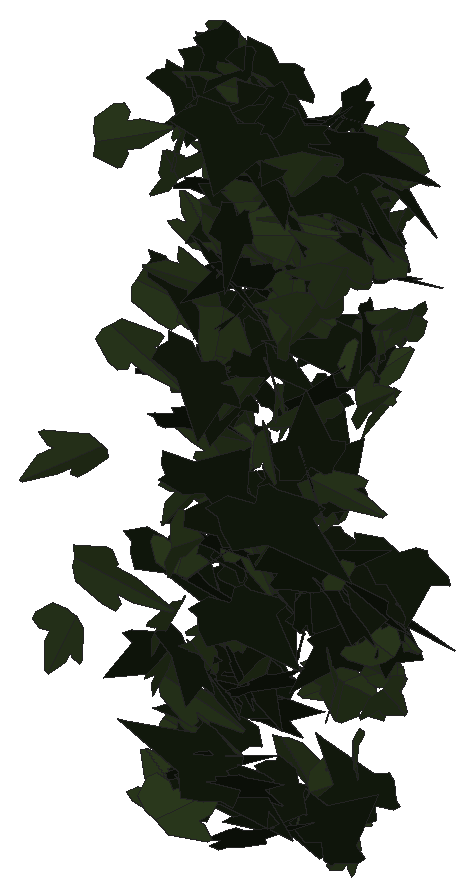
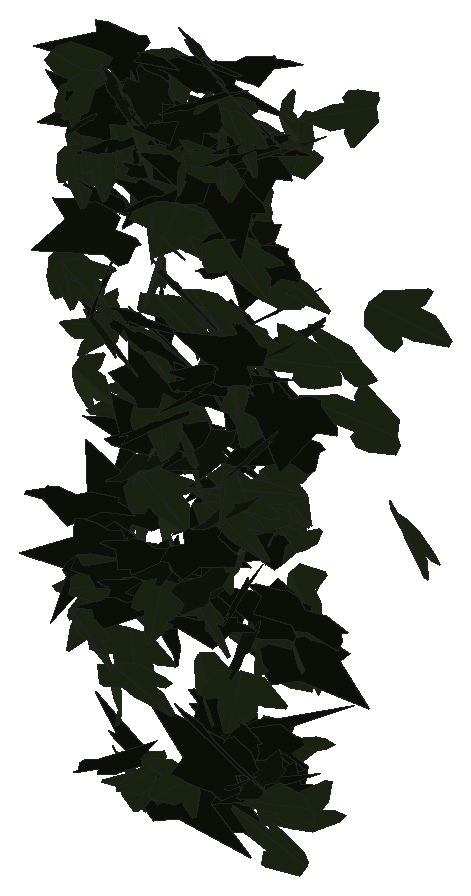
# SketchUp Ruby script. Lengths in millimetres.
U = 1.mm
M = Sketchup.active_model
def pt(a) = Geom::Point3d.new(a.map { |v| v * U })
def face(e, loops, mat)
  f = e.add_face(loops[0].map { |a| pt(a) })
  loops[1..].each { |l| e.add_face(l.map { |a| pt(a) }).erase! }
  f.material = f.back_material = mat if mat
  f
end
# faces: each face lists its corners as indices into pts; further lists are holes
def faces(e, pts, list, mat = nil) = list.each { |f| face(e, (f[0].is_a?(Array) ? f : [f]).map { |l| l.map { |i| pts[i] } }, mat) }
# xy, xz, yz: faces in a plane at the given z, y or x. An outline is a flat list of corners, or four numbers for a rectangle; further outlines are holes
def ring(l) = l.size == 4 ? [[l[0], l[1]], [l[2], l[1]], [l[2], l[3]], [l[0], l[3]]] : l.each_slice(2).to_a
def flat(e, list, mat, &to3) = list.each { |f| face(e, (f[0].is_a?(Array) ? f : [f]).map { |l| ring(l).map { |u, v| to3.(u, v) } }, mat) }
def xy(e, z, list, mat = nil) = flat(e, list, mat) { |x, y| [x, y, z] }
def xz(e, y, list, mat = nil) = flat(e, list, mat) { |x, z| [x, y, z] }
def yz(e, x, list, mat = nil) = flat(e, list, mat) { |y, z| [x, y, z] }
def lines(e, pts, list) = list.each { |a, b| e.add_line(pt(pts[a]), pt(pts[b])) }
# prism: a flat outline (further loops are holes) pulled along v
def prism(e, loops, v, mat = nil)
  f = face(e, loops, mat); d = Geom::Vector3d.new(v.map { |x| x * U })
  f.pushpull(f.normal.samedirection?(d) ? d.length : -d.length)
end
def box(e, o, s, mat = nil) = prism(e, [[o, [o[0] + s[0], o[1], o[2]], [o[0] + s[0], o[1] + s[1], o[2]], [o[0], o[1] + s[1], o[2]]]], [0, 0, s[2]], mat)
def at(x, y, z, deg = 0) = Geom::Transformation.translation(pt([x, y, z])) * Geom::Transformation.rotation(ORIGIN, Z_AXIS, deg.degrees)
def axes(o, x, y, z) = Geom::Transformation.new([*x, 0, *y, 0, *z, 0, *pt(o).to_a, 1])
def part(name) = M.definitions.add(name)
# library, detail: a bought-in or finely detailed component or shape, given as its bounding box
def library(name, o, s) = part(name).tap { |d| box(d.entities, o, s) }
def detail(e, o, s) = box(e.add_group.entities, o, s)
def put(e, d, t, mat = nil) = e.add_instance(d, t).tap { |i| i.material = mat if mat }
def group(e, t, mat = nil) = e.add_group.tap { |g| g.transformation = t; g.material = mat if mat }.entities
root = M.entities
M.materials.add("efeu1").color = [18, 25, 13]
M.materials.add("efeu2").color = [43, 57, 29]
c1 = part("ivyleaf_10")
p = [[0,12.8,-0.8],[-1.5,51.3,-10.9],[-4.9,51,-11.6],[-13.6,26.5,-7.3],[-13.2,15.9,-4.6],[-21.1,19.3,-7.2],
  [-29.5,16.3,-8.3],[-29.2,8.3,-6.2],[-19.7,-9.8,0.5],[-7.6,-13,4],[1,-12.2,5.8],[-0.4,51.1,-11.1],
  [-1.5,51.1,-10.9],[1,-12.4,5.9],[16.9,-12.4,3.5],[35.1,9.1,-5.1],[35,12.9,-6.1],[20.5,16.4,-4.9],
  [15.8,15,-3.8],[15.3,27.6,-7.1],[12.8,31.3,-7.8]]
faces(c1.entities,p,[[0,1,2,3,4,5,6,7,8,9,10],[11,12,0,13,14,15,16,17,18,19,20]],"efeu2")
c2 = part("ivyleaf_9")
p = [[39.1,54.8,31.7],[34.5,51.8,30.2],[-5.3,25.2,17.3],[-17.9,28.3,20.9],[-21.6,21.7,17],[-20.2,4.3,5.3],
  [-22.9,-0.3,2.5],[-17.1,-4,-0.6],[-2,-2.1,-1.2],[-0.7,-15.4,-10.1],[16.6,-22.3,-16.7],[21.1,-15.1,-12.5],
  [32.7,-10.7,-11],[46.1,-1.8,-6.6],[30.8,11.2,3.8]]
faces(c2.entities,p,[[0,1,2,3,4,5,6,7,8,9,10,11,12,13,14]],"efeu1")
put(root,c1,axes([3953.5,539.1,2196.3],[-0.45606,-0.68527,1.0215],[-0.63132,-0.96615,-0.72595],[2.25434,-0.4092,0.00335]))
put(root,c1,axes([3962.8,543.3,2043.3],[0.10342,-0.11388,1.24145],[2.36353,0.11376,-0.04392],[-0.20776,1.23742,0.11829]))
put(root,c1,axes([3909.3,561.1,1942.6],[1.68125,-0.86872,0.00346],[0.02052,0.00603,-1.23891],[1.65324,0.88336,0.01186]))
put(root,c2,axes([4068.5,665.6,1979.6],[0.04124,-0.63779,-0.98844],[0.0507,0.98862,-0.63733],[2.23826,-0.01064,0.03265]))
put(root,c1,axes([3895,656.8,2533.3],[0.07259,-0.06329,-1.22483],[1.29662,1.02007,-0.03149],[1.94096,-0.67907,0.06685]))
put(root,c2,axes([4052.5,691.4,2465.4],[-1.13162,0.14311,-0.93716],[1.64141,-0.37766,-0.60485],[-0.74915,-1.04364,0.09037]))
put(root,c2,axes([3994.6,700.6,2252.2],[-0.32323,-1.18488,0.38736],[-0.17032,-0.37834,-1.19653],[2.36639,-0.18908,-0.03321]))
put(root,c2,axes([4159.4,697.8,2148],[-0.25535,0.03617,1.01376],[-0.12285,-1.02082,0.02788],[1.9267,-0.06029,0.13614]))
put(root,c2,axes([4097.7,676.6,2113.9],[0.01123,-0.60676,-1.09595],[0.88147,1.01936,-0.56186],[2.21521,-0.40255,0.22913]))
put(root,c1,axes([3970.5,669.2,1675.2],[1.18753,0.16446,-0.9582],[1.172,0.81418,0.54075],[1.4318,-0.80286,0.3521]))
put(root,c2,axes([3966.8,711,1862.7],[-0.11397,-0.83575,0.70239],[-0.09588,-0.70059,-0.83789],[2.07554,-0.07825,-0.00014]))
put(root,c2,axes([4035,713.2,2571.4],[-1.13596,-0.94572,0.0103],[0.01136,-0.01595,-1.11824],[1.79996,-0.59674,0.01356]))
put(root,c1,axes([3948.4,708.4,1913.9],[0.23071,-1.13641,0.33175],[0.13111,-0.32615,-1.14239],[2.24927,0.13558,0.03256]))
put(root,c1,axes([3949,717.6,2475.8],[-0.50415,-0.86215,-0.63928],[-0.37326,-0.60849,0.9019],[-2.00833,0.32952,-0.00715]))
put(root,c1,axes([3948.5,712,1812.2],[0.14236,-0.098,1.21389],[2.30428,-0.12512,-0.08471],[0.24986,1.20974,0.08957]))
put(root,c1,axes([4190.8,709.8,2458.3],[-1.59618,-0.19977,0.58892],[-1.03173,-0.24965,-0.85669],[0.57996,-0.99393,0.09681]))
put(root,c2,axes([3992.8,704.3,1985],[0.50189,0.92298,0.30225],[-0.18514,-0.28652,0.95981],[1.83911,-0.28072,0.01414]))
put(root,c1,axes([4185.4,711.9,2432.1],[-1.3066,-0.76689,0.17145],[-0.19512,-0.13831,-1.02918],[1.4828,-0.69397,0.01565]))
put(root,c1,axes([4110.9,699.4,2073.7],[-0.11913,-0.98771,-0.66786],[0.13344,0.66457,-0.98942],[2.26527,-0.09109,0.02316]))
put(root,c1,axes([3940,714,1849.5],[0.2568,-1.17504,0.03833],[0.00608,-0.03822,-1.18276],[2.23752,0.13496,-0.00118]))
put(root,c1,axes([3871.8,712.3,2237.8],[1.0563,0.08963,0.93672],[1.77529,0.09088,-0.56138],[-0.23596,1.085,-0.03036]))
put(root,c2,axes([4117.5,694.3,2028.2],[0.38673,0.0841,1.23687],[2.17532,0.47271,-0.21991],[-0.91378,1.1609,-0.00006]))
put(root,c2,axes([4001.8,728.5,1715.6],[-0.69414,-1.1102,-0.37263],[-0.21997,-0.35426,1.16857],[-2.21789,0.3826,0.00073]))
put(root,c1,axes([4113.7,692.7,2334.9],[0.23097,0.0758,-1.11438],[0.23761,1.11299,0.0893],[2.11247,-0.13348,0.1118]))
put(root,c2,axes([3990.1,714.2,2080.1],[-1.10932,-0.03055,0.83181],[1.54238,-0.25252,0.5586],[0.36144,0.98381,0.16921]))
put(root,c1,axes([4138.1,723.1,2372.2],[-1.11874,-1.08665,0.27018],[-0.24108,-0.23865,-1.23545],[2.11739,-0.60131,0.00209]))
put(root,c1,axes([4185.8,699.1,1902.9],[0.38525,-0.55887,-1.09726],[-0.1788,1.10174,-0.57848],[2.33675,0.17644,0.13664]))
put(root,c1,axes([3958.5,697.5,2007.9],[0.02773,-0.40498,-1.16165],[0.39577,1.14583,-0.39685],[2.30766,-0.19165,0.08202]))
put(root,c2,axes([4068.5,700.4,1861.9],[0.97182,0.67719,0.56864],[0.59009,0.47784,-0.84747],[-1.5761,0.59645,0.03333]))
put(root,c1,axes([4054.8,736.4,2159.7],[0.47293,-0.25048,0.96234],[1.33711,-0.65777,-0.35262],[1.33937,0.74511,0.01222]))
put(root,c1,axes([3941.5,737.7,2536.9],[0.70975,-0.78141,0.76922],[0.69407,-0.67784,-0.86539],[1.96804,0.52086,0.02779]))
put(root,c2,axes([4165.7,746.5,1982.1],[-0.19574,-0.69461,0.89319],[0.21233,-0.89873,-0.68607],[2.14296,0.0256,0.14956]))
put(root,c2,axes([4030.4,722.8,2058.2],[-1.5828,0.55974,0.19008],[-0.30204,0.10464,-1.00247],[-1.08374,-0.84666,0.00177]))
put(root,c2,axes([4036.3,734.5,2378.4],[-0.27964,0.51781,-0.87248],[-0.03773,-0.88288,-0.52065],[-1.93057,-0.05775,0.13655]))
put(root,c1,axes([4032,732.8,2225.2],[-0.46898,-0.95582,0.27345],[-0.13208,-0.2645,-0.98707],[1.88749,-0.256,-0.00113]))
put(root,c1,axes([3986.1,733.5,2418.8],[0.08471,-0.20955,0.99847],[1.9016,-0.19306,-0.08506],[0.39247,0.98064,0.19662]))
put(root,c2,axes([3931.7,736.4,1846.1],[0.21674,0.29858,-0.99083],[-0.63281,-0.93341,-0.31949],[-1.86509,0.35139,-0.00674]))
put(root,c2,axes([4011.5,714.2,1707.4],[1.50908,0.55786,0.29525],[0.44153,0.18329,-0.96937],[-1.11716,0.82601,0.0157]))
put(root,c2,axes([4142.6,713.4,2170],[-1.68294,0.61344,-0.33012],[-0.53232,0.17594,1.07612],[1.21427,0.92734,0.01421]))
put(root,c2,axes([4041.8,752.3,2497.9],[-0.10021,-0.90569,0.67551],[0.45221,-0.67,-0.87977],[2.10226,0.10095,0.22144]))
put(root,c1,axes([4131.1,737.3,2547.4],[-1.06216,-0.86661,0.25518],[-0.27664,-0.20989,-1.03073],[1.69694,-0.57665,-0.00831]))
put(root,c1,axes([3944.9,719.4,1970.1],[0.62125,0.76329,-0.56949],[0.42362,0.52419,0.83016],[1.76228,-0.39509,0.00121]))
put(root,c1,axes([3964.5,723.6,1865.7],[-0.87576,-0.9413,-0.64512],[0.46835,0.59738,-1.04716],[2.12073,-0.52063,-0.03515]))
put(root,c1,axes([3954.2,748.1,2064.2],[-0.264,-1.04651,0.60457],[-0.14105,-0.60003,-1.05565],[2.29586,-0.1572,0.00466]))
put(root,c2,axes([3976.3,745.6,2366.7],[0.92675,-0.82806,0.32776],[0.27851,-0.29408,-0.96038],[1.67189,0.508,-0.0217]))
put(root,c1,axes([3978.4,744.7,2134.1],[-1.15558,0.06455,0.81247],[1.47221,-0.27349,0.59981],[0.48859,0.97672,0.11426]))
put(root,c1,axes([4152.6,728.8,2020.2],[1.45952,-0.41695,0.66634],[-1.04669,0.38051,0.87104],[-1.06885,-0.94198,0.05691]))
put(root,c1,axes([4095.5,740.5,2439.4],[1.21864,-0.81411,-0.13122],[-0.1254,0.11509,-1.03557],[1.56439,0.6434,0.01921]))
put(root,c1,axes([3968,735.6,2332.1],[-0.45998,0.05211,0.98861],[-1.88399,0.00032,-0.24202],[-0.02414,-1.01773,0.05054]))
put(root,c1,axes([4067.1,731.7,2433.4],[0.74237,-0.07838,-0.94898],[1.76944,0.25294,0.36126],[0.39159,-0.99435,0.1667]))
put(root,c1,axes([4058.2,754.4,2215.6],[-0.58744,0.37768,0.92115],[1.15732,-0.69208,0.48752],[1.50025,0.68177,-0.0154]))
put(root,c2,axes([4070.7,746.8,2593.4],[-1.58531,0.49418,-0.33539],[0.45174,-0.25427,-0.96413],[-1.04305,-0.86121,0.0922]))
put(root,c2,axes([3950.7,725.8,1702.5],[0.48371,0.7736,-0.6093],[0.23986,0.59854,0.81251],[1.85875,-0.27856,0.05372]))
put(root,c2,axes([3980.4,750.8,2204.1],[-1.5148,-0.23059,-0.56353],[1.05969,0.09972,-0.82721],[0.46898,-0.97012,0.04892]))
put(root,c2,axes([3984.6,738.2,1699.9],[-0.34655,-0.27365,-1.02257],[1.17235,0.81643,-0.32817],[1.63841,-0.64207,0.01853]))
put(root,c2,axes([4095.1,757,2572.2],[-1.6129,-0.6342,-0.07722],[0.09986,0.05876,-1.05838],[1.21181,-0.84895,-0.01557]))
put(root,c1,axes([4011.9,755,2009.1],[1.36658,-0.30645,0.80688],[1.44018,-0.28134,-0.78025],[0.79014,1.04283,0.02661]))
put(root,c1,axes([4018.3,741.9,2389.7],[-0.05518,-0.93369,-0.40921],[0.0848,0.40782,-0.93368],[1.93831,-0.04442,0.0292]))
put(root,c2,axes([4000.7,736.6,1619.8],[0.81016,0.88116,-0.3023],[0.25031,0.27219,0.97859],[1.75521,-0.44554,-0.00002]))
put(root,c1,axes([3925.2,750,1636.4],[1.02843,1.0486,0.35028],[-0.33649,-0.3029,1.17951],[2.07702,-0.56828,0.01765]))
put(root,c1,axes([4084.4,744,2450.3],[-1.39093,-0.35841,-0.61342],[1.05352,0.26436,-0.81398],[0.84755,-0.9168,0.00509]))
put(root,c2,axes([4066,773.8,2463.1],[0.04859,-0.91032,0.80064],[0.13213,-0.79841,-0.90999],[2.30349,0.065,0.03531]))
put(root,c2,axes([4074.1,758.7,2565.5],[-1.83403,0.05238,0.56183],[-1.06917,0.01546,-0.96499],[-0.10096,-1.11537,0.01301]))
put(root,c2,axes([3970.6,749.5,1650.7],[-1.55831,-0.63423,0.4677],[0.70388,0.28629,1.03569],[-1.32434,0.89844,0.00014]))
put(root,c2,axes([3971,748.9,1996.1],[1.92699,-0.01233,-0.06006],[-0.11401,0.01285,-1.0125],[0.02487,1.0142,0.0121]))
put(root,c1,axes([4045.2,740.9,2017],[-0.78325,0.56329,0.78885],[-0.84278,0.6531,-0.69737],[-1.64106,-0.60426,-0.01837]))
put(root,c2,axes([4007,764.4,2069.1],[0.31794,-0.9687,-0.45375],[-0.0926,0.4519,-0.98265],[2.03375,0.17201,0.0262]))
put(root,c2,axes([4124.7,759,2513.7],[-0.10012,-0.49736,-0.98113],[1.02595,0.84456,-0.45703],[1.82488,-0.5021,0.20311]))
put(root,c1,axes([3961.6,771.5,2266.6],[2.04598,-0.563,0.17863],[0.32051,-0.06341,-1.21333],[1.07749,1.08792,0.02172]))
put(root,c2,axes([3921.5,750.9,2138.8],[1.51379,0.4763,0.35874],[0.59959,0.1721,-0.927],[-0.96353,0.85541,-0.01324]))
put(root,c1,axes([4127.6,759.7,2116.8],[-0.99301,-0.24041,-0.78625],[1.42432,0.24674,-0.57207],[0.64798,-0.91079,0.05256]))
put(root,c2,axes([4145.5,756.5,2564.8],[0.48075,0.11841,-0.99049],[1.0605,0.83074,0.24142],[1.57471,-0.59561,0.13981]))
put(root,c2,axes([4140.8,783.3,1909.8],[-0.17794,0.32339,-1.06895],[0.56755,-1.02651,-0.33663],[-2.04831,-0.31252,-0.00041]))
put(root,c2,axes([3913.1,775.4,1911.4],[0.89855,-0.42368,0.70592],[1.1409,-0.38089,-0.62953],[1.07405,0.75905,0.07813]))
put(root,c2,axes([4117.1,769.5,1645.8],[-0.82484,0.76744,0.77397],[0.73898,-0.66955,0.88133],[1.93829,0.58185,-0.00665]))
put(root,c1,axes([4040.8,794.5,2388.6],[-0.00111,-0.21122,1.13229],[-0.12037,-1.13057,-0.21093],[2.18884,-0.06228,-0.01103]))
put(root,c2,axes([4134.4,787.4,1969.5],[2.07397,-0.28345,-0.41835],[0.77322,-0.09994,1.12597],[-0.57192,-1.16298,0.0052]))
put(root,c2,axes([3976,762.5,2499.1],[0.51319,0.98217,-0.04078],[-0.03108,-0.03781,-1.0185],[-1.87063,0.27008,0.00573]))
put(root,c2,axes([3887.1,790.5,2292.9],[0.13252,-0.96869,0.27036],[0.07949,-0.26799,-0.97094],[1.91241,0.07826,0.02162]))
put(root,c2,axes([3917.3,765.1,2191.8],[1.20879,0.83868,-0.24486],[-0.31172,-0.18307,-1.05185],[-1.63333,0.65562,0.01953]))
put(root,c1,axes([3948.4,773.4,2225.4],[1.29995,-0.65518,0.33657],[-0.47755,0.22459,0.9464],[-1.318,-0.72758,-0.01094]))
put(root,c2,axes([4166.6,798.5,1982],[-0.50155,-0.92701,0.44825],[-0.13821,-0.44481,-0.9626],[1.95483,-0.26929,0.04695]))
put(root,c1,axes([3941.4,772.5,2048.7],[-0.10233,-0.07689,-1.07137],[2.00959,0.193,-0.06684],[0.37502,-1.05522,0.06584]))
put(root,c2,axes([4013.8,761.7,2211],[-0.13756,0.46618,0.92228],[-0.42672,0.89543,-0.47018],[-1.91992,-0.23242,0.03842]))
put(root,c2,axes([3909.3,799.8,2535.7],[-0.63465,-0.89236,0.41066],[0.08578,-0.44712,-0.93499],[1.86758,-0.28271,0.1825]))
put(root,c2,axes([4126.9,795.4,2483.9],[0.47542,-0.14624,-1.14518],[2.12427,-0.2688,0.2778],[-0.56144,-1.14087,0.08134]))
put(root,c2,axes([4018.8,798.9,1913],[0.15359,-0.88599,0.51674],[0.25457,-0.50481,-0.88645],[1.93539,0.13671,0.07559]))
put(root,c2,axes([4053.2,800.8,1682],[-0.54873,-0.7516,0.52577],[-0.38099,-0.48629,-0.80494],[1.70363,-0.35084,-0.01066]))
put(root,c1,axes([4145.2,781.7,1646.1],[1.09834,-0.74826,-0.2803],[-0.31591,0.22596,-0.94494],[1.48756,0.60046,0.00629]))
put(root,c1,axes([3953.9,777.5,2187.9],[-1.15627,-0.84557,-0.34477],[0.3323,0.2989,-1.04074],[1.70585,-0.63137,-0.03096]))
put(root,c2,axes([3879.1,787.1,1942.1],[-0.67637,-0.36584,-0.94495],[1.60956,0.4445,-0.49016],[1.06228,-0.90645,0.14102]))
put(root,c1,axes([4096.2,776.3,1988],[0.28382,-0.9081,-0.59435],[-0.26561,0.57891,-0.91952],[2.04841,0.20089,-0.03688]))
put(root,c2,axes([3983.9,785,2288.3],[-0.97506,0.78708,-0.34025],[0.39122,-0.27206,-0.93886],[-1.58435,-0.55157,-0.02243]))
put(root,c1,axes([4177.5,795.2,1907.3],[0.2415,0.91034,0.6083],[-0.20402,-0.5991,0.91893],[2.07375,-0.16496,0.01957]))
put(root,c2,axes([4087.7,778.2,2081.4],[-1.10349,-0.08986,0.99776],[1.8689,0.17722,0.5866],[-0.37741,1.14031,-0.01254]))
put(root,c2,axes([4114.9,796.2,2421.9],[-1.74984,-0.0918,-0.41817],[0.78731,0.06471,-0.92375],[0.20991,-1.00798,-0.02122]))
put(root,c2,axes([3966.6,806.4,2529.1],[-1.20519,-0.47169,0.62719],[-0.99407,-0.34815,-0.7892],[1.1147,-0.82046,-0.02569]))
put(root,c1,axes([3865.8,781.8,2266.7],[0.56961,0.1229,1.15898],[1.94317,0.54939,-0.32192],[-1.06968,1.06347,0.03237]))
put(root,c1,axes([4205.3,781.5,2435.1],[0.14544,-0.09058,-1.08147],[-1.61418,0.6714,-0.11617],[1.28862,0.85125,-0.02346]))
put(root,c2,axes([4127,795.9,1919.8],[0.17776,-0.00701,1.13133],[-2.05606,0.33653,0.09128],[-0.63938,-1.08415,0.02102]))
put(root,c1,axes([3995.9,794,2030.2],[1.42057,-0.17644,-0.64816],[-1.17648,0.19882,-0.76598],[0.50038,0.96836,0.03917]))
put(root,c1,axes([4093.4,813,2057.9],[-0.51625,0.49807,1.00316],[0.66044,-0.94399,0.56253],[2.02668,0.43449,0.07222]))
put(root,c2,axes([4084.7,781.8,1914.3],[-0.26341,-0.30348,0.95173],[0.92118,0.82013,0.33191],[-1.66313,0.50233,0.0331]))
put(root,c1,axes([4167.3,776.1,2231.5],[-0.07976,-0.2334,-1.06216],[0.47707,1.03225,-0.23672],[2.014,-0.25376,0.01401]))
put(root,c2,axes([4149.1,805.6,2495.8],[-1.76884,0.07374,0.34309],[-0.66787,-0.19852,-0.90795],[0.00222,-0.97061,0.21177]))
put(root,c2,axes([4068.4,798.9,1647.5],[0.20727,0.10245,-1.06024],[-1.6467,-0.6131,-0.14812],[-1.1824,0.87182,0.02042]))
put(root,c1,axes([4113.2,811.5,2476.4],[-0.24081,-0.87466,0.44632],[0.24827,-0.461,-0.86643],[1.85229,-0.05192,0.17416]))
put(root,c2,axes([4132.2,803.1,2502.2],[-0.51447,-0.84002,-0.601],[0.30844,0.57905,-0.88223],[1.94142,-0.3146,-0.0191]))
put(root,c2,axes([4099.6,805.5,2558.9],[-0.97737,0.70542,-0.56719],[0.35998,-0.55409,-0.86038],[-1.68468,-0.52765,0.14521]))
put(root,c1,axes([3963.1,804.7,2076.7],[0.78458,0.27682,0.93431],[-1.62873,-0.38233,0.49088],[0.88696,-0.94694,0.07493]))
put(root,c1,axes([3931.4,800.3,2348.3],[1.68288,0.19811,0.41243],[-0.7633,-0.09632,0.90614],[0.41911,-0.97092,-0.00574]))
put(root,c1,axes([4187.5,803.1,2516.9],[-0.96599,-0.88923,-0.05619],[0.06294,0.04582,-1.02387],[1.69459,-0.5086,0.006]))
put(root,c1,axes([3989.1,806.9,2558],[0.38613,0.05653,-1.1268],[-2.14688,-0.01,-0.20361],[-0.03781,1.14487,0.05386]))
put(root,c1,axes([4123.1,821.9,1746.2],[-0.05872,-0.04989,-0.93839],[0.28043,-0.92754,0.04447],[-1.76635,-0.1456,0.03826]))
put(root,c1,axes([4204.7,805.2,2555.2],[0.79101,0.00843,-0.96101],[-1.78295,0.2372,-0.40308],[0.40816,1.01981,0.1017]))
put(root,c2,axes([4081.6,820.5,2465.8],[-1.70627,-0.38907,0.27039],[-0.46015,-0.12199,-0.9772],[0.77549,-0.92844,0.01509]))
put(root,c1,axes([4079.3,815.4,2046.4],[-0.96799,-0.78369,0.47894],[-0.49743,-0.40134,-0.93427],[1.67572,-0.57184,-0.00067]))
put(root,c1,axes([4006.4,805.3,1828.6],[-0.00174,-1.13497,-0.31256],[0.0126,0.31255,-1.13496],[2.24045,-0.00264,0.00614]))
put(root,c1,axes([4089.7,807.4,1653.3],[1.12223,0.71891,0.1206],[0.14571,0.09319,-0.9298],[-1.37968,0.5946,-0.0001]))
put(root,c1,axes([4119.7,806,1826.2],[-1.97486,0.08011,0.28638],[-0.54346,0.02176,-1.04074],[-0.15798,-1.07622,0.00027]))
put(root,c1,axes([3879.6,804.7,1693.5],[0.45792,0.142,0.90249],[1.53877,0.40146,-0.27872],[-0.80961,0.84334,-0.01928]))
put(root,c2,axes([3931.5,831.1,1884.3],[0.62047,-0.31201,-1.00483],[1.42929,-0.66778,0.45101],[-1.4025,-0.81856,0.01508]))
put(root,c1,axes([4180.8,801.3,1845.6],[-0.39427,-0.80324,-0.61711],[0.44774,0.5745,-0.82676],[1.87508,-0.30608,0.06766]))
put(root,c1,axes([3873.9,819.5,1637.3],[0.5582,-0.21869,-1.04088],[1.67761,-0.55426,0.36483],[-1.13281,-0.92858,0.02738]))
put(root,c2,axes([4137.3,817,2253.6],[-1.29238,0.26166,0.62516],[-1.27255,-0.11437,-0.67841],[-0.2103,-0.91589,0.26332]))
put(root,c2,axes([3948,831.8,1938.3],[-0.17983,-0.23298,0.97162],[-0.68537,-0.90242,-0.25141],[1.7738,-0.3723,0.00136]))
put(root,c2,axes([3964.1,830.1,2382.7],[-1.09507,-0.5983,0.55719],[-0.76726,-0.38512,-0.82985],[1.35368,-0.70228,-0.01961]))
put(root,c2,axes([3948.5,820,2596],[-1.70653,0.26347,-0.4856],[0.83738,-0.21931,-0.93142],[-0.63591,-0.99585,0.07665]))
put(root,c2,axes([4063.8,816.1,2178.6],[1.1598,0.75277,0.57103],[-0.67247,-0.44863,0.96849],[1.66776,-0.70439,-0.00659]))
put(root,c1,axes([4021.6,805.3,2482.3],[-1.18871,0.31001,0.74421],[-1.38088,0.19425,-0.68985],[-0.66889,-0.95196,0.10159]))
put(root,c2,axes([3958.8,804.3,1803.2],[1.13108,-0.36565,-0.72433],[-1.15541,0.39529,-0.69766],[1.02453,0.84946,0.01287]))
put(root,c2,axes([4057.8,796.8,1852.4],[0.02798,0.06476,1.01548],[0.47963,0.98371,-0.06638],[-1.87625,0.25244,-0.00183]))
put(root,c2,axes([4000.2,833,2584.9],[-0.68689,-0.94212,0.23799],[-0.08422,-0.23767,-1.00799],[1.84744,-0.36112,0.04253]))
put(root,c2,axes([3973.1,803.8,2523.5],[1.26364,-0.11037,0.7519],[1.37575,0.39986,-0.57962],[-0.44638,0.91994,0.34215]))
put(root,c1,axes([3969.8,807.7,1973.1],[-0.4208,0.82835,-0.48441],[-0.3427,0.45246,0.8559],[1.79386,0.28075,0.04988]))
put(root,c2,axes([4158.9,824,2517.9],[1.03256,-0.88522,-0.02887],[-0.02657,0.0253,-1.03825],[1.68543,0.54272,0.00132]))
put(root,c2,axes([4168.4,824.1,2406.1],[-1.64668,0.22294,0.41903],[-0.81337,0.01313,-0.88942],[-0.39301,-0.96126,0.08503]))
put(root,c2,axes([3992.8,833.5,2547.9],[0.64634,-0.77266,0.60737],[0.6546,-0.50853,-0.83924],[1.75218,0.475,0.08949]))
put(root,c2,axes([4133,841.2,2296.1],[0.28206,-0.311,-1.0442],[1.42462,-0.73667,0.32565],[-1.50673,-0.75474,0.11243]))
put(root,c1,axes([4139.9,822.1,2518.7],[-1.62721,-0.49771,0.25526],[-0.4485,-0.10234,-0.98887],[0.96547,-0.88639,-0.02916]))
put(root,c1,axes([4071.3,808.7,2334.1],[0.39779,-0.71741,-0.74078],[0.29983,0.76919,-0.70047],[1.9396,0.02823,0.26021]))
put(root,c2,axes([4062,842.1,1941.5],[0.10819,-0.55444,0.98982],[0.38287,-0.97043,-0.55513],[2.12501,0.20308,0.04962]))
put(root,c1,axes([4138,816.8,1890.5],[-1.55676,-0.47877,-0.41518],[0.69427,0.1986,-0.94771],[0.98622,-0.89555,0.01179]))
put(root,c1,axes([3978.2,822.4,2405.1],[1.16531,-0.02497,-0.8142],[-1.53435,0.12723,-0.61017],[0.22193,1.01076,0.05669]))
put(root,c2,axes([3933.3,843,1711],[-0.04755,-0.79926,-0.70561],[-0.03794,-0.70533,0.79965],[-2.02876,0.03192,0.00159]))
put(root,c1,axes([4061.2,822.7,2161.7],[-0.84814,-1.10077,-0.12168],[0.06919,0.11655,-1.18752],[2.10662,-0.44701,-0.00998]))
put(root,c2,axes([4174.9,833.3,2008.4],[-1.10334,-0.74969,-0.43056],[0.57691,0.30922,-0.94657],[1.54093,-0.65257,0.0461]))
put(root,c1,axes([4137.6,812.8,2497.7],[-0.26906,0.99957,-0.54875],[-0.12347,0.545,1.00946],[2.16669,0.15518,-0.01062]))
put(root,c2,axes([3949.7,834.7,1796.6],[-0.71936,-0.16034,-0.92484],[1.75075,0.13495,-0.39935],[0.35518,-0.98994,0.09536]))
put(root,c2,axes([3911.5,831.9,2562.3],[0.12425,-0.94013,-0.42619],[0.14037,0.4302,-0.93768],[1.95951,0.0288,0.09419]))
put(root,c2,axes([3985.8,838.6,1912.2],[-1.03709,-0.74016,-0.17178],[0.1777,0.14456,-0.91906],[1.43515,-0.55276,-0.01033]))
put(root,c1,axes([4128.4,839.2,2278.6],[1.33501,-0.65634,0.53358],[0.78177,-0.34165,-0.96025],[1.4073,0.81242,0.02725]))
put(root,c2,axes([4127.9,818.9,2411.3],[-1.0909,0.66557,0.53877],[-0.61776,0.43107,-0.87785],[-1.50809,-0.65803,-0.03013]))
put(root,c2,axes([4070.2,847.4,2084.7],[-0.27746,-0.8937,0.45989],[0.14809,-0.47335,-0.89517],[1.90714,-0.09327,0.13642]))
put(root,c2,axes([3967.4,821.3,2225.3],[0.75166,-0.62505,-0.72425],[-0.14774,0.76002,-0.69825],[1.81474,0.32077,0.24314]))
put(root,c2,axes([4127.5,827.4,1942.5],[1.63875,-0.30925,0.40015],[0.73703,-0.10497,-0.91443],[0.61902,0.94367,0.02942]))
put(root,c2,axes([4122,842.6,2521.3],[0.5076,-0.44193,0.88519],[0.91454,-0.74354,-0.51599],[1.64598,0.54941,0.01372]))
put(root,c2,axes([3920.5,817.1,2414.1],[1.08608,0.82522,-0.07792],[-0.10426,-0.05684,-1.00323],[-1.57409,0.57314,0.01269]))
put(root,c1,axes([4153.2,821.7,2549.9],[-0.70675,-0.69007,-0.62037],[0.76792,0.48164,-0.77729],[1.59034,-0.53924,0.09963]))
put(root,c1,axes([4039.3,832.8,2305.8],[1.63363,-0.01865,-0.46369],[-0.88037,0.04369,-0.85805],[0.07072,0.97462,0.02959]))
put(root,c1,axes([3940,827.4,1840.9],[-1.29819,-0.81872,-0.27806],[0.34392,0.21137,-1.06562],[1.60926,-0.70563,0.00343]))
put(root,c1,axes([4098.1,826.4,1918.1],[-1.3645,-0.04182,-0.99963],[1.89586,0.08489,-0.718],[0.17764,-1.22722,-0.01561]))
put(root,c2,axes([4177.7,816.1,1910],[0.27257,-0.1899,-1.0038],[-1.08906,0.82477,-0.23768],[1.61068,0.58981,0.00917]))
put(root,c1,axes([3991.2,827.8,2322.6],[1.50794,-0.30631,-0.63638],[-0.94173,0.44166,-0.82865],[0.95911,0.91525,0.18689]))
put(root,c2,axes([4067.9,832.1,1921.1],[-0.46936,-0.51909,-0.74662],[0.69863,0.65092,-0.57381],[1.58336,-0.44108,0.03186]))
put(root,c1,axes([4070.7,813.6,1678.3],[-0.13063,-0.16482,-1.07537],[0.70969,1.00867,-0.1784],[1.94511,-0.37909,-0.00713]))
put(root,c2,axes([3980.8,819.7,2478.4],[0.01288,-0.02086,1.06759],[1.80848,0.48712,0.00349],[-0.92702,0.95001,0.02165]))
put(root,c2,axes([4102.1,840.5,2500.6],[-0.07943,-0.99592,-0.39194],[0.06339,0.39083,-0.99667],[2.03595,-0.05102,0.01574]))
put(root,c2,axes([3964.3,827.4,2483.8],[1.15291,0.21239,-0.79905],[-1.51017,-0.12896,-0.63584],[-0.4421,0.99439,0.0882]))
put(root,c1,axes([4009,820.7,2510],[0.03317,0.78359,0.64214],[-0.40413,0.6308,-0.76398],[-1.88529,-0.12143,0.17507]))
put(root,c1,axes([4174.2,835.6,2450.6],[-0.42614,-1.02151,-0.09899],[0.02772,0.09814,-1.04574],[1.95304,-0.22428,-0.00675]))
put(root,c1,axes([4171.4,846.1,2306.7],[-0.86961,-0.70836,0.4892],[-0.21962,-0.49844,-0.82953],[1.62362,-0.44682,0.14981]))
put(root,c1,axes([4137.8,815.1,2234],[0.74753,0.28681,-1.10408],[0.97667,0.99844,0.44193],[1.93893,-0.61351,0.20306]))
put(root,c2,axes([4132.8,839.1,1669.5],[-1.22223,-0.77018,0.1958],[0.26711,0.13786,1.00261],[-1.48865,0.65707,0.01914]))
put(root,c1,axes([4068,830,2412.1],[0.41654,-0.81272,-0.55175],[-0.04479,0.56078,-0.83535],[1.869,0.19457,0.10295]))
put(root,c1,axes([3938.7,835.2,2253.8],[0.03257,-0.9549,-0.29214],[0.07101,0.29259,-0.95418],[1.89918,0.00544,0.04069]))
put(root,c2,axes([4051.3,843.1,1984.6],[-0.71882,-0.66772,-0.64977],[0.79765,0.50442,-0.76198],[1.58366,-0.55714,0.08886]))
put(root,c1,axes([4013.3,842.5,1695.4],[-1.35655,0.49616,-0.50103],[0.69758,-0.34789,-0.86595],[-1.14644,-0.79878,0.06594]))
put(root,c2,axes([4043.8,843.2,2448.5],[0.16728,-0.93191,-0.4056],[-0.07174,0.40384,-0.93605],[1.93299,0.09564,0.00036]))
put(root,c1,axes([4028.9,836,2427.3],[-1.53689,-0.55281,-0.28257],[0.44319,0.16006,-0.97863],[1.09533,-0.84044,-0.00051]))
put(root,c2,axes([4114.2,844.6,2572.6],[-1.33295,0.55446,-0.49499],[0.75188,-0.29839,-0.89322],[-1.1982,-0.80405,-0.00985]))
put(root,c2,axes([4130.2,824.6,2368.3],[1.69058,0.23998,0.34562],[0.43651,0.4007,-0.86771],[-0.67137,0.86483,0.30613]))
put(root,c2,axes([3938.2,844.9,1735.1],[1.8419,0.04784,-0.53455],[0.97537,0.24487,0.94976],[0.30326,-1.07815,0.19199]))
put(root,c1,axes([3960.8,832.5,2542.7],[0.55702,-0.75201,-0.67991],[-0.07308,0.69894,-0.78959],[1.92807,0.24374,0.1665]))
put(root,c1,axes([4068.5,840.6,2253.1],[1.39621,-0.49173,-0.51728],[-0.75146,0.33834,-0.88158],[1.13153,0.83144,0.05281]))
put(root,c2,axes([3989.7,857.7,2237.3],[-0.76947,-0.76048,-0.65377],[-0.58865,-0.57599,0.86127],[-1.81563,0.50904,-0.00217]))
put(root,c1,axes([4090.3,847.5,1811.4],[1.45769,0.01934,-0.58414],[-1.1123,0.01621,-0.76577],[-0.01054,0.96311,0.02462]))
put(root,c2,axes([3993.3,831.9,1761],[-0.84246,0.65901,0.74542],[-0.77081,0.62587,-0.79382],[-1.72963,-0.59991,-0.00931]))
put(root,c2,axes([3877.6,860.8,1748.4],[0.36845,-0.71401,0.58022],[0.29804,-0.5587,-0.73978],[1.72546,0.24897,0.00389]))
put(root,c1,axes([4141.7,859.8,2188.7],[0.25357,-0.79902,0.62138],[0.12879,-0.61831,-0.80957],[1.9221,0.14684,-0.02773]))
put(root,c2,axes([3933.8,865.8,2077.9],[-0.37421,-0.82672,0.54571],[0.01013,-0.55723,-0.84226],[1.88526,-0.16111,0.11284]))
put(root,c1,axes([3949.9,851.8,2525],[-1.09637,0.12856,-0.81085],[1.32198,-0.45171,-0.5651],[-0.83291,-0.88617,0.17042]))
put(root,c1,axes([4007.8,841.9,2140.8],[0.73772,-0.90079,-0.45227],[-0.32834,0.41812,-0.98063],[1.89004,0.42424,0.00618]))
put(root,c1,axes([4157.7,841.5,1852.7],[1.02413,-0.55875,-0.58439],[-0.75242,0.43051,-0.77566],[1.34229,0.66764,0.01108]))
put(root,c1,axes([3985.4,837.9,1926.3],[0.71085,-0.46335,-0.72167],[-0.78571,0.5928,-0.59427],[1.43066,0.55579,0.0322]))
put(root,c2,axes([3987.6,863,2022.6],[-0.18922,0.03829,-0.96352],[0.30964,-0.95408,-0.0547],[-1.80891,-0.16732,0.09143]))
put(root,c1,axes([4179.3,847.5,2317.9],[-0.41705,-0.97227,-0.07492],[0.04772,0.07114,-0.99662],[1.85529,-0.22038,0.00879]))
put(root,c2,axes([4137.5,851.1,2263.1],[-1.4244,0.52503,-0.45128],[0.71204,-0.25245,-0.91419],[-1.10865,-0.83669,-0.00734]))
put(root,c2,axes([3951,850.2,2151.9],[1.14023,-0.76727,-0.08514],[-0.08066,0.07492,-0.97339],[1.46702,0.60048,0.01266]))
put(root,c1,axes([4131.5,846.1,2480.2],[-0.38203,-1.02151,-0.18149],[0.03157,0.18167,-1.04088],[1.97433,-0.20057,-0.01848]))
put(root,c1,axes([4072.4,849,2526],[0.4555,-0.98114,-0.10103],[-0.03854,0.09905,-1.00991],[1.87679,0.24016,0.00378]))
put(root,c2,axes([3908.6,858.1,2283.5],[0.91039,-0.53882,0.69882],[0.85714,-0.53449,-0.7204],[1.44423,0.65687,-0.01296]))
put(root,c1,axes([3930.5,843.5,2585.2],[1.38526,-0.56503,-0.47277],[-0.40862,0.47305,-0.89592],[1.34128,0.72767,0.21533]))
put(root,c2,axes([3893.8,841.5,2175.1],[1.04154,-0.5114,-0.69257],[-0.66213,0.61929,-0.7322],[1.49876,0.62898,0.15782]))
put(root,c1,axes([4038.8,845.4,1933.3],[-0.80147,-0.96534,-0.41897],[0.37335,0.37135,-1.05279],[1.9677,-0.46365,0.0291]))
put(root,c2,axes([4082.1,856.6,1909.6],[-0.48128,-0.85343,-0.45675],[0.37061,0.41757,-0.88804],[1.80457,-0.31337,0.06057]))
put(root,c2,axes([3957.4,863.4,1972.1],[0.6839,-0.8808,0.28544],[0.16221,-0.27342,-0.95099],[1.75469,0.36857,-0.02334]))
put(root,c2,axes([3909.9,861.9,2560.4],[-0.17202,-0.99865,-0.13127],[0.14254,0.12477,-1.00076],[1.91167,-0.09916,0.06281]))
put(root,c1,axes([3944.1,842.8,2108.8],[0.01644,-0.791,-0.58161],[0.16967,0.57986,-0.7873],[1.86086,-0.04588,0.07692]))
put(root,c2,axes([4062.9,860.7,2270],[-1.74929,-0.08867,-0.348],[0.66868,-0.02419,-0.92181],[0.1414,-0.98251,0.0541]))
put(root,c1,axes([3929.1,854.3,2422.4],[-1.59235,-0.21288,0.52401],[-0.91156,-0.23101,-0.85858],[0.57256,-0.95981,0.09042]))
put(root,c2,axes([4006.7,836.7,2327.2],[-1.27487,0.89332,-0.01825],[-0.02742,0.012,1.11656],[1.7003,0.67,0.00432]))
put(root,c2,axes([4031,858,2167.1],[0.2112,-0.97649,-0.29116],[0.03652,0.29483,-0.98149],[1.93896,0.10081,0.0502]))
